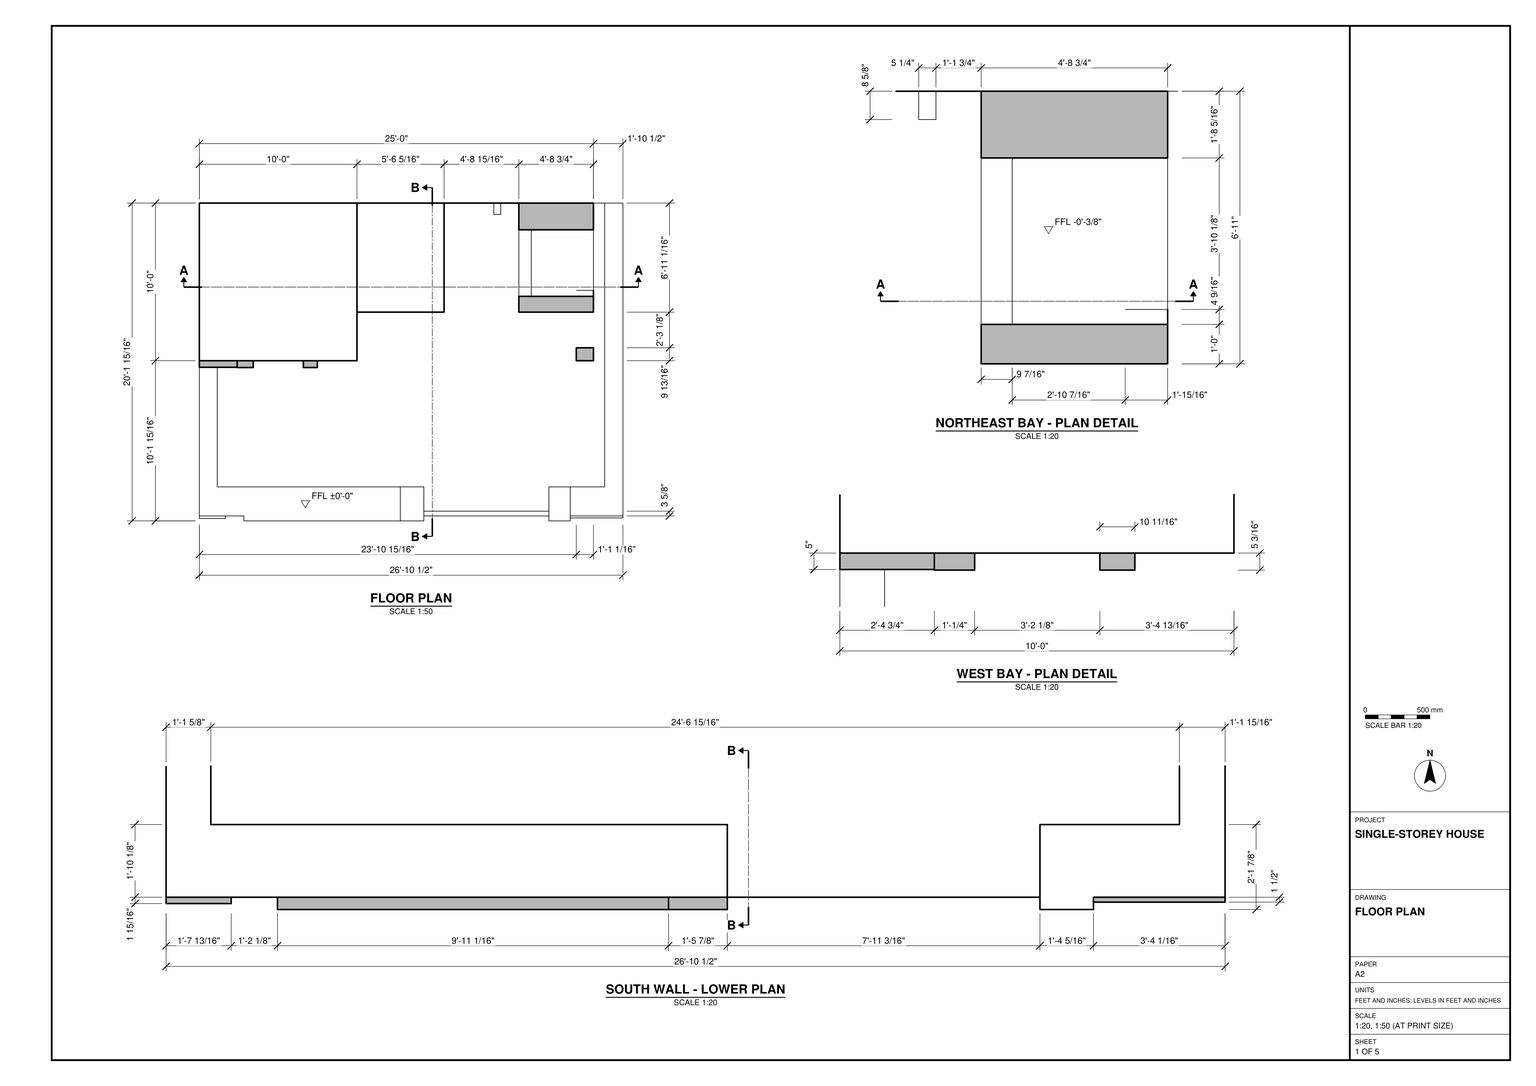
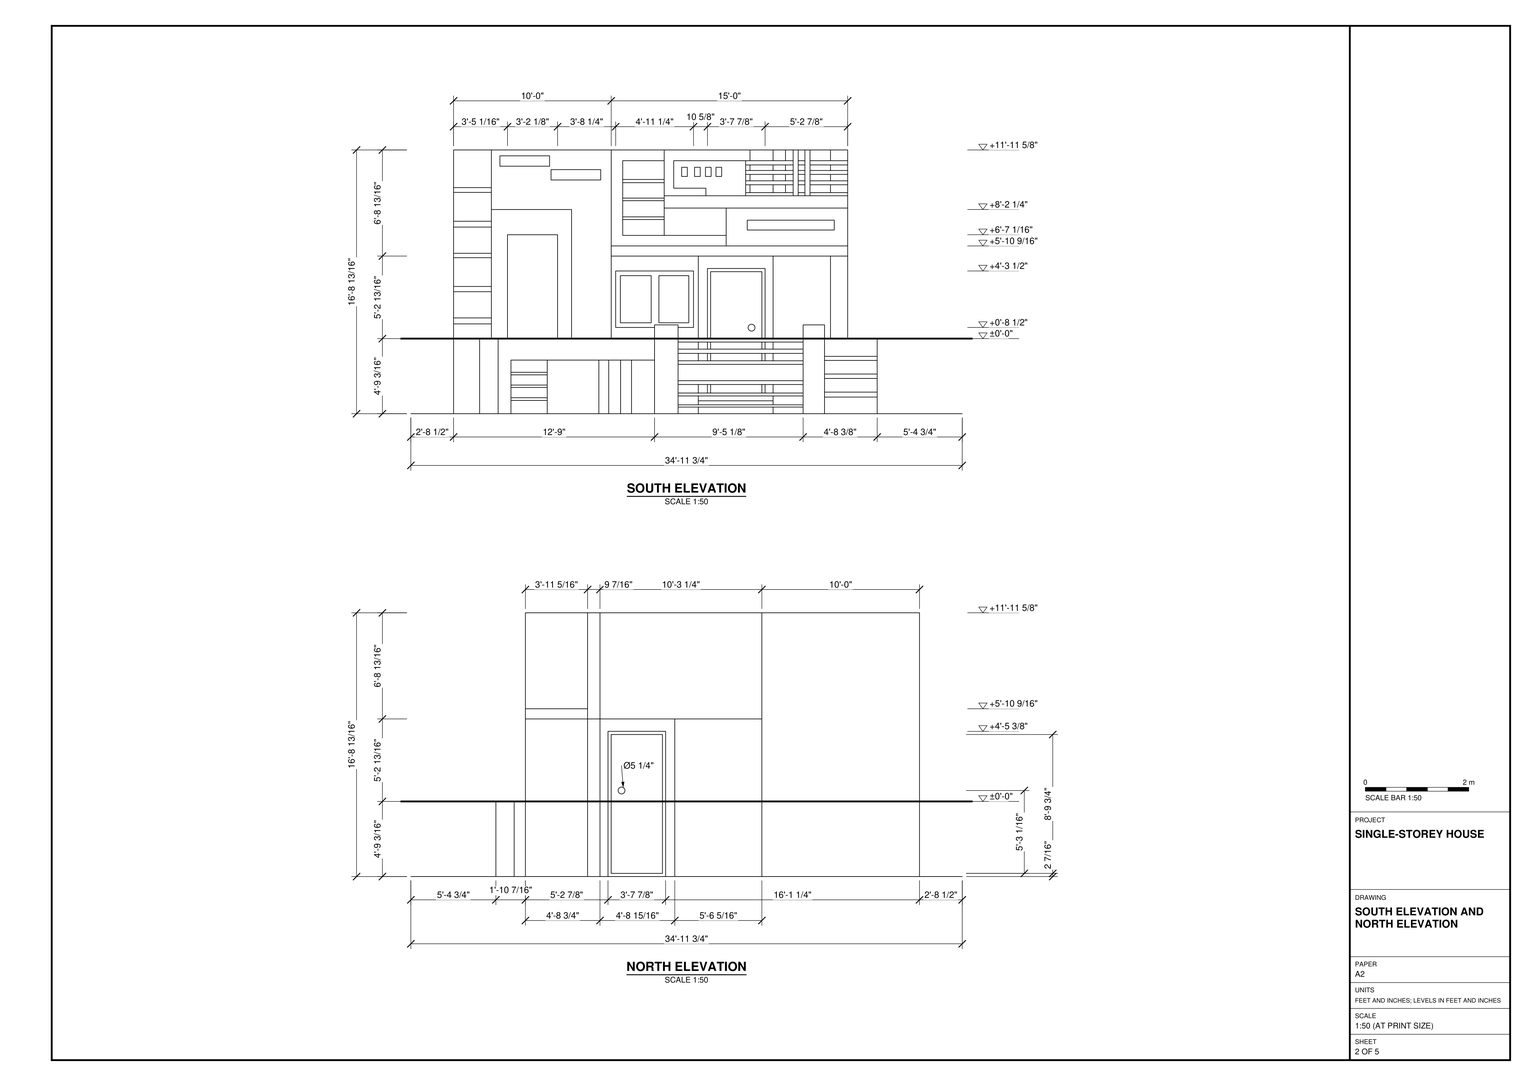
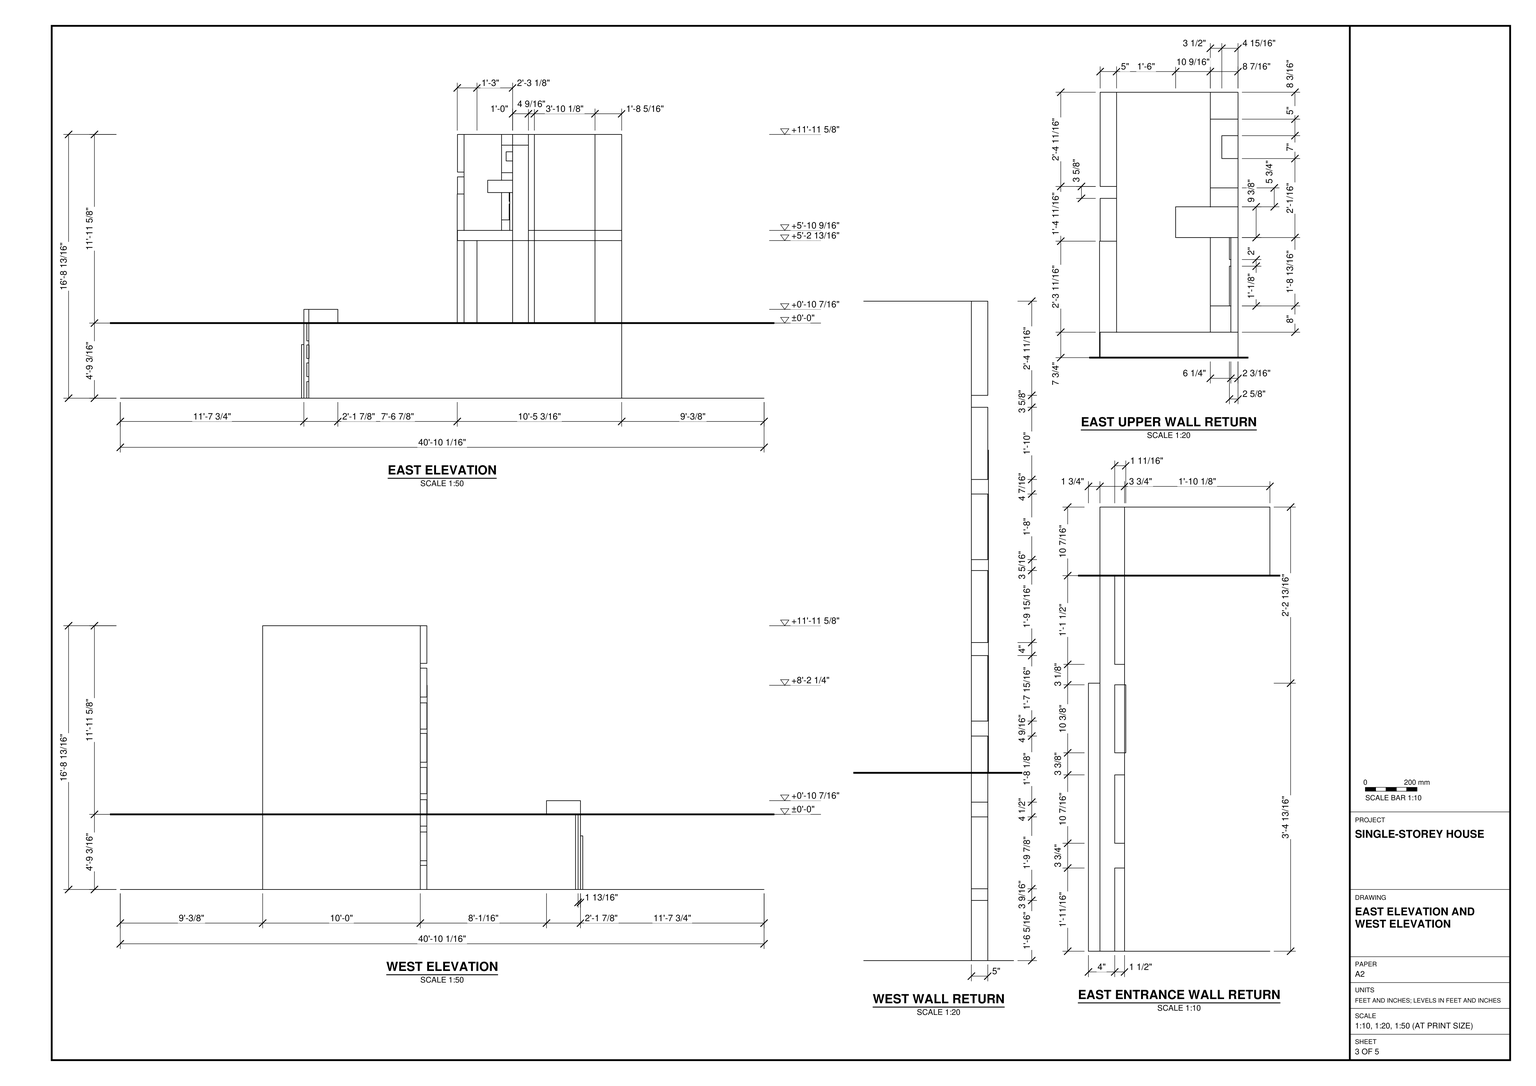
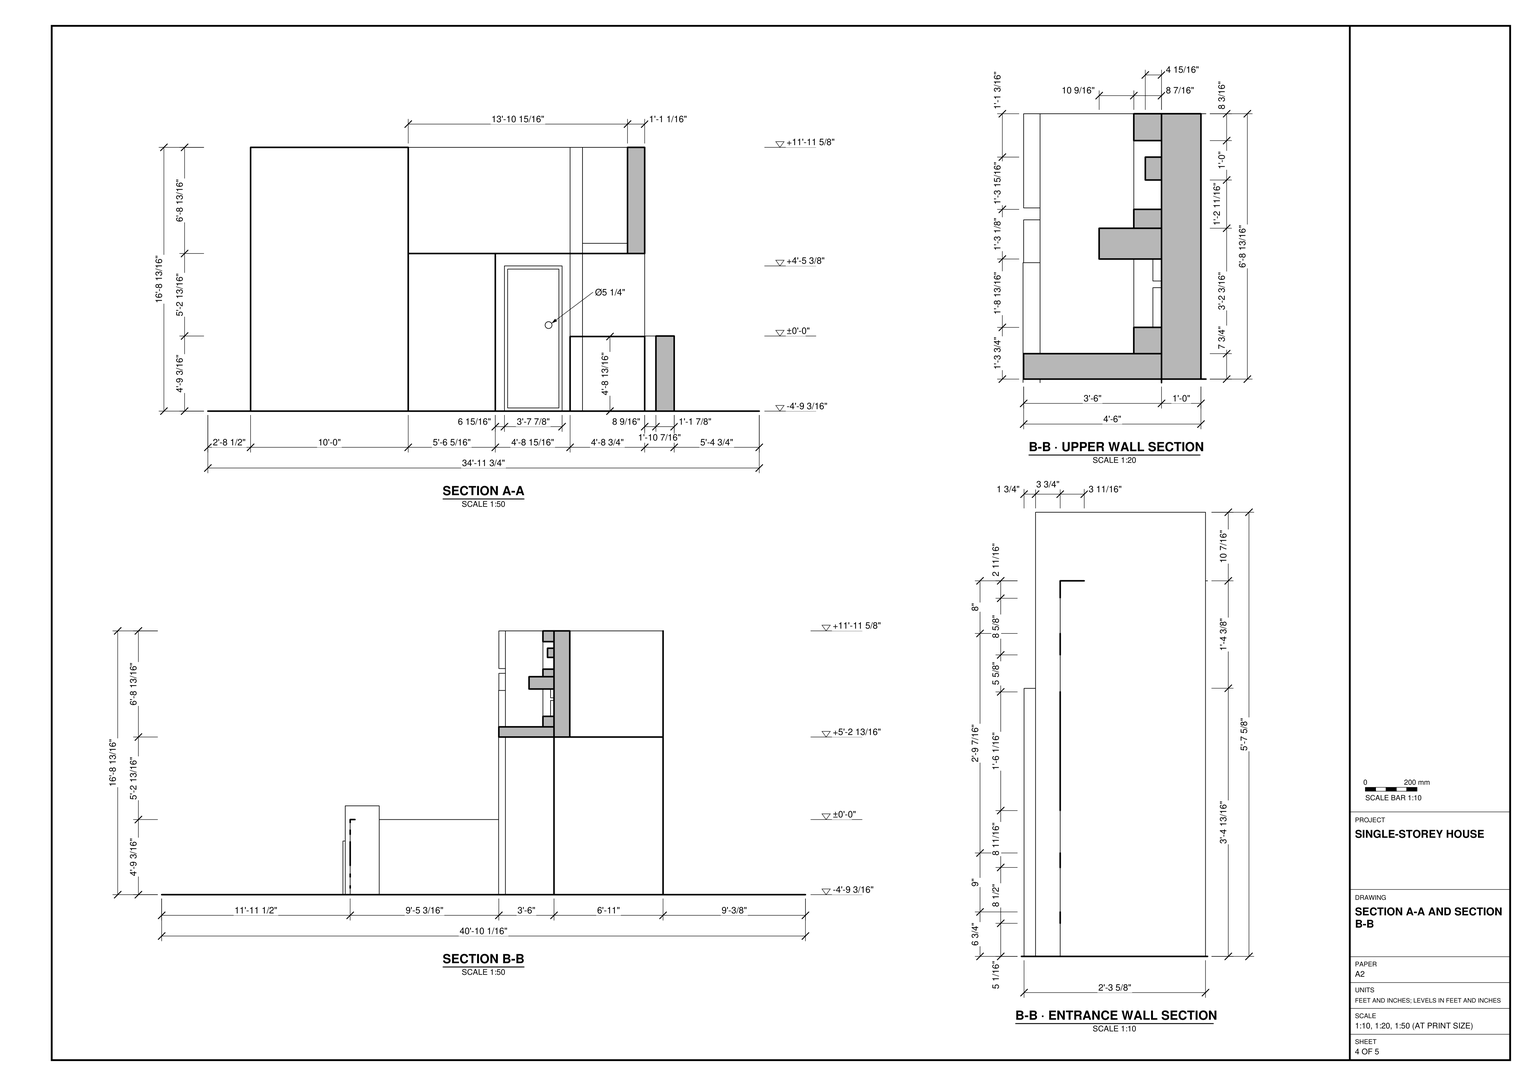
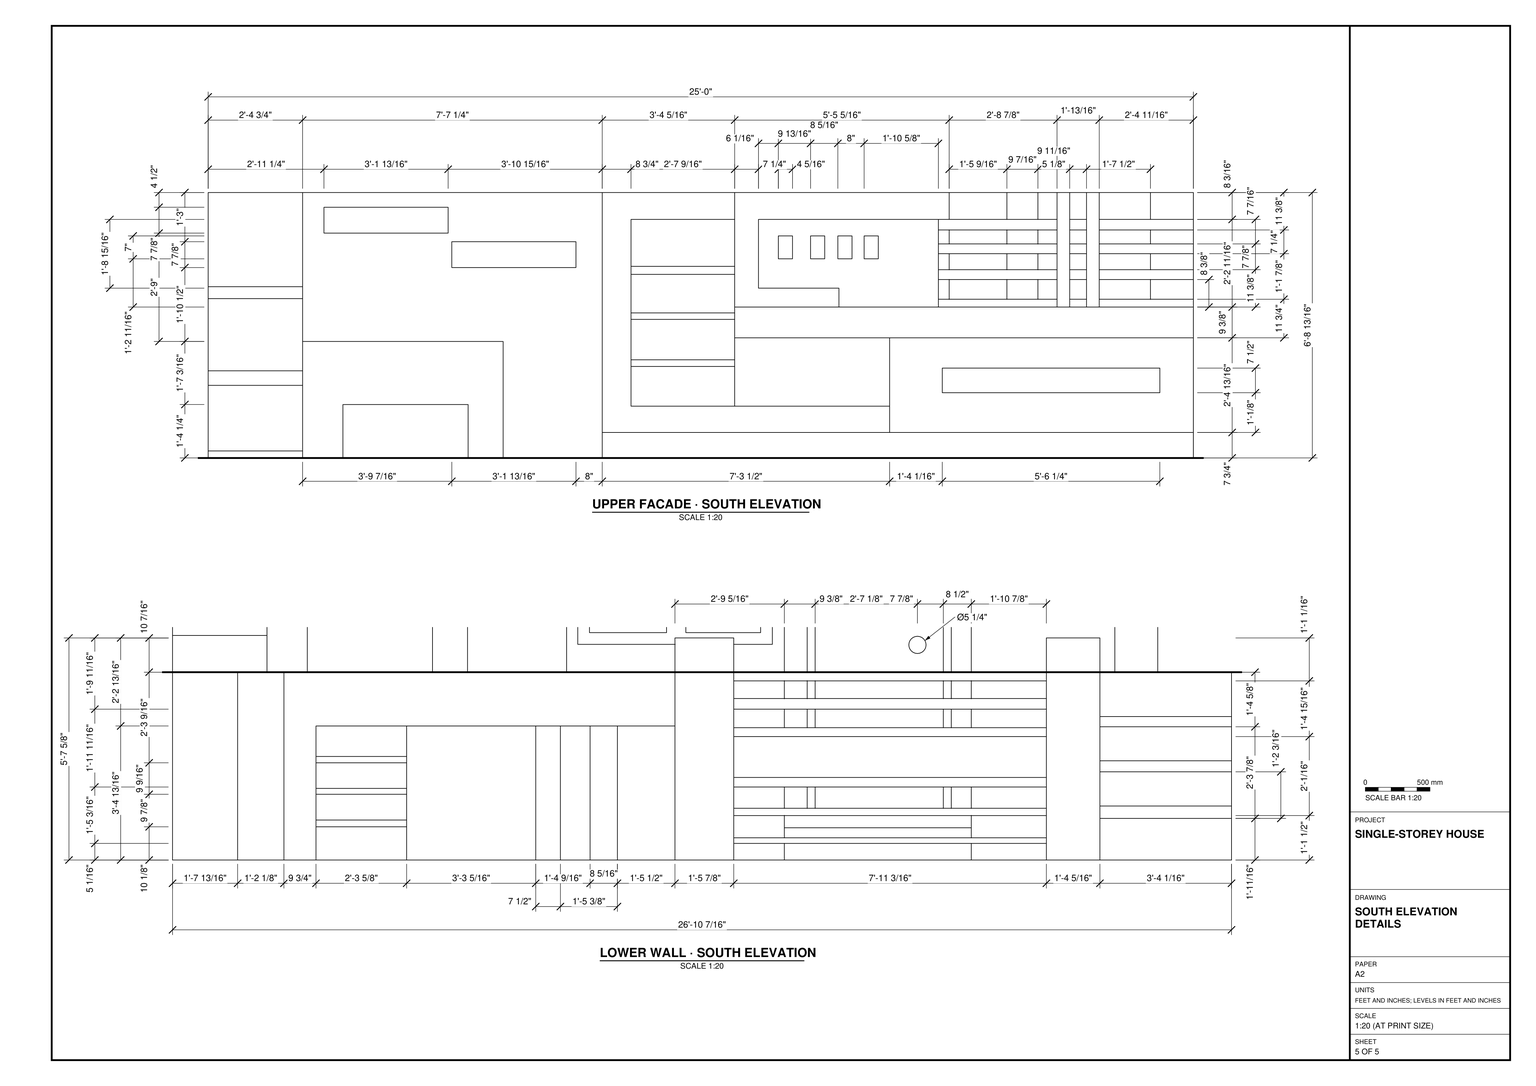
Build the single-storey house in SketchUp from task_files/diagram_01.pdf. Work in feet and inches. The complete model measures 34'-11 3/4" along X, 40'-10 1/16" along Y and 16'-8 13/16" along Z. Use ±0'-0" as the finished floor level. The overall height includes geometry below this datum; it is not the height of the wall above the floor.

Set out the square west bay, the shallower adjoining bay and the narrow northeast bay from the floor plan. Leave the forecourt between the house and the south entrance wall. Follow the plan details for wall thicknesses and returns, and match the slab and roof edges to the drawings. On the south facade, place the divided window beside the entrance door. Model the tall rectangular framing on the west side and the bands and panels above the openings on the east side. Use the side elevations to determine how far these details project. Build the lower entrance wall with its posts and horizontal slats.

Keep the walls, slabs and roof separate as groups or components. Keep each furniture or joinery piece shown separate and use components for repeated parts. Any decor or loose items shown may be represented by suitable library components. Save one SketchUp model as output_files/single_storey_house_and_its_south_entrance_wall.skp.

# SketchUp Ruby script. Lengths in inches.
U = 1.inch
M = Sketchup.active_model
def pt(a) = Geom::Point3d.new(a.map { |v| v * U })
def face(e, loops, mat)
  f = e.add_face(loops[0].map { |a| pt(a) })
  loops[1..].each { |l| e.add_face(l.map { |a| pt(a) }).erase! }
  f.material = f.back_material = mat if mat
  f
end
# faces: each face lists its corners as indices into pts; further lists are holes
def faces(e, pts, list, mat = nil) = list.each { |f| face(e, (f[0].is_a?(Array) ? f : [f]).map { |l| l.map { |i| pts[i] } }, mat) }
# xy, xz, yz: faces in a plane at the given z, y or x. An outline is a flat list of corners, or four numbers for a rectangle; further outlines are holes
def ring(l) = l.size == 4 ? [[l[0], l[1]], [l[2], l[1]], [l[2], l[3]], [l[0], l[3]]] : l.each_slice(2).to_a
def flat(e, list, mat, &to3) = list.each { |f| face(e, (f[0].is_a?(Array) ? f : [f]).map { |l| ring(l).map { |u, v| to3.(u, v) } }, mat) }
def xy(e, z, list, mat = nil) = flat(e, list, mat) { |x, y| [x, y, z] }
def xz(e, y, list, mat = nil) = flat(e, list, mat) { |x, z| [x, y, z] }
def yz(e, x, list, mat = nil) = flat(e, list, mat) { |y, z| [x, y, z] }
def lines(e, pts, list) = list.each { |a, b| e.add_line(pt(pts[a]), pt(pts[b])) }
# prism: a flat outline (further loops are holes) pulled along v
def prism(e, loops, v, mat = nil)
  f = face(e, loops, mat); d = Geom::Vector3d.new(v.map { |x| x * U })
  f.pushpull(f.normal.samedirection?(d) ? d.length : -d.length)
end
def box(e, o, s, mat = nil) = prism(e, [[o, [o[0] + s[0], o[1], o[2]], [o[0] + s[0], o[1] + s[1], o[2]], [o[0], o[1] + s[1], o[2]]]], [0, 0, s[2]], mat)
def at(x, y, z, deg = 0) = Geom::Transformation.translation(pt([x, y, z])) * Geom::Transformation.rotation(ORIGIN, Z_AXIS, deg.degrees)
def axes(o, x, y, z) = Geom::Transformation.new([*x, 0, *y, 0, *z, 0, *pt(o).to_a, 1])
def part(name) = M.definitions.add(name)
# library, detail: a bought-in or finely detailed component or shape, given as its bounding box
def library(name, o, s) = part(name).tap { |d| box(d.entities, o, s) }
def detail(e, o, s) = box(e.add_group.entities, o, s)
def put(e, d, t, mat = nil) = e.add_instance(d, t).tap { |i| i.material = mat if mat }
def group(e, t, mat = nil) = e.add_group.tap { |g| g.transformation = t; g.material = mat if mat }.entities
root = M.entities
M.materials.add("[0006_Pink]").color = [255, 192, 203]
M.materials.add("[0017_IndianRed]").color = [205, 92, 92]
M.materials.add("[0063_GreenYellow]").color = [173, 255, 47]
M.materials.add("[0087_Cyan]").color = [0, 255, 255]
M.materials.add("[0108_Indigo]").color = [75, 0, 130]
M.materials.add("[0110_LightSlateGray]").color = [119, 136, 153]
M.materials.add("[0119_RosyBrown]").color = [188, 143, 143]
M.materials.add("[Brick Colored Blue]1").color = [144, 143, 146]
M.materials.add("[Metal Seamed]").color = [118, 119, 115]
M.materials.add("[Translucent Glass Gray]").color = [128, 128, 128]
M.materials["[Translucent Glass Gray]"].alpha = 0.5
M.materials.add("[Wood Lumber ButtJoined]").color = [164, 152, 112]
M.materials.add("[Wood Veneer 01]").color = [120, 70, 37]
xy(root,0,[[203.42,123.43,298.62,143.5],[143.13,138,150.63,143.5],[159.68,138,167.99,143.5],[66.45,139.75,76.21,143.5],[185.52,139.75,203.42,143.5],
  [298.62,139.75,314.92,143.5],[76.21,141.125,103.82,143.5],[32.53,141.5625,52.35,143.5],[314.92,142,354.99,143.5],[32.53,143.5,32.53,256.6875,46.15,256.6875,46.15,165.625,203.42,165.625,203.42,143.5],
  [203.42,143.5,203.42,165.625,46.15,165.625,46.15,256.6875,61.29,256.6875,61.29,256.5,73.57,256.5,73.57,261.6875,111.69,261.6875,111.69,256.5,122.36,256.5,122.36,261.6875,152.53,261.6875,152.53,298.67,218.83,298.67,218.83,244.42,275.75,244.42,275.75,298.67,332.53,298.67,332.53,271.53,319.47,271.53,319.47,261.6875,332.53,261.6875,332.53,381.6875,341.09,381.6875,341.09,165.625,298.62,165.625,298.62,143.5],[298.62,143.5,298.62,165.625,341.09,165.625,341.09,381.6875,354.99,381.6875,354.99,143.5],[218.83,244.42,275.75,261.61],[61.29,256.5,73.57,261.6875],[111.69,256.5,122.36,261.6875],
  [32.53,256.6875,46.15,261.6875],[46.15,256.6875,61.29,261.6875],[218.83,261.61,275.75,278.81],[32.53,261.6875,152.53,381.6875],[319.47,261.6875,332.53,271.53],
  [218.83,278.81,275.75,298.67],[152.53,298.67,218.83,381.6875],[218.83,298.67,275.75,381.6875],[275.75,298.67,285.2,381.6875],[285.2,298.67,285.2,381.6875,332.53,381.6875,332.53,315.23,319.47,315.23,319.47,298.67],
  [319.47,298.67,332.53,315.23]])
xy(root,0,[[[0,0,419.74,490.0625],[218.83,244.42,275.75,244.42,275.75,298.67,332.53,298.67,332.53,381.6875,32.53,381.6875,32.53,256.6875,61.29,256.6875,61.29,256.5,73.57,256.5,73.57,261.6875,111.69,261.6875,111.69,256.5,122.36,256.5,122.36,261.6875,152.53,261.6875,152.53,298.67,218.83,298.67],[203.42,123.43,298.62,123.43,298.62,139.75,314.92,139.75,314.92,142,354.99,142,354.99,381.6875,341.09,381.6875,341.09,165.625,298.62,165.625,298.62,143.5,185.52,143.5,185.52,139.75,203.42,139.75],[319.47,261.6875,332.53,271.53],[66.45,139.75,76.21,139.75,76.21,141.125,103.82,141.125,103.82,143.5,66.45,143.5],[159.68,138,167.99,143.5],[143.13,138,150.63,143.5],[32.53,141.5625,52.35,143.5]]],"[Brick Colored Blue]1")
xy(root,5.5,[[218.83,244.42,275.75,261.61]])
xy(root,9.8125,[[218.83,261.61,275.75,278.81]])
xy(root,10.11,[[76.21,141.125,103.82,143.5]])
xy(root,12.17,[[76.21,141.125,103.82,143.5]])
xy(root,12.67,[[314.92,142,354.99,143.5]])
xy(root,14.375,[[218.83,278.81,275.75,298.67]])
xy(root,16.4375,[[314.92,142,354.99,143.5]])
xy(root,18.33,[[32.53,256.6875,61.29,261.6875]])
xy(root,20.01,[[76.21,141.125,103.82,143.5]])
xy(root,21.8,[[76.21,141.125,103.82,143.5]])
xy(root,21.88,[[32.53,256.6875,61.29,261.6875]])
xy(root,26.85,[[314.92,142,354.99,143.5]])
xy(root,29.6,[[76.21,141.125,103.82,143.5]])
xy(root,30.21,[[314.92,142,354.99,143.5],[314.92,143.5,354.99,143.6875]])
xy(root,31.53,[[76.21,141.125,103.82,143.5]])
xy(root,40.57,[[314.92,142,354.99,143.5],[314.92,143.5,354.99,143.6875]])
xy(root,40.8125,[[143.13,138,150.63,139.75],[159.68,138,167.99,139.75],[143.13,139.75,150.63,143.5],[159.68,139.75,167.99,143.5],[76.21,141.125,103.82,143.5]])
xy(root,40.8125,[[76.21,139.75,103.82,141.125],[103.82,139.75,143.13,143.5],[150.63,139.75,159.68,143.5],[167.99,139.75,185.52,143.5]],"[0087_Cyan]")
xy(root,43.68,[[314.92,142,354.99,143.5]])
xy(root,43.77,[[32.53,256.6875,61.29,261.6875]])
xy(root,48.26,[[32.53,256.6875,61.29,261.6875]])
xy(root,56.8125,[[275.75,310.68,285.2,361.37],[285.2,310.68,332.53,361.37]],"[0006_Pink]")
xy(root,57.1875,[[66.45,139.75,185.52,143.5],[314.92,142,354.99,143.5],[32.53,143.5,185.52,143.5,185.52,165.625,46.15,165.625,46.15,256.6875,32.53,256.6875],[314.92,143.5,354.99,143.5,354.99,381.6875,341.09,381.6875,341.09,165.625,314.92,165.625]])
xy(root,57.1875,[[32.53,141.5625,52.35,143.5]],"[0108_Indigo]")
xy(root,57.1875,[[203.42,143.5,298.62,147.15]],"[Metal Seamed]")
xy(root,67.625,[[185.52,139.75,203.42,143.5],[298.62,139.75,314.92,165.625],[185.52,143.5,203.42,165.625]],"[0108_Indigo]")
xy(root,68.38,[[32.53,256.6875,61.29,261.6875]])
xy(root,72.95,[[32.53,256.6875,61.29,261.6875]])
xy(root,92.9,[[32.53,256.6875,61.29,261.6875]])
xy(root,96.87,[[32.53,256.6875,61.29,261.6875]])
xy(root,118.79,[[32.53,256.6875,61.29,261.6875]])
xy(root,120,[[319.47,261.6875,332.53,271.53],[152.53,298.67,218.83,310.68],[275.75,298.67,285.2,310.68],[285.2,298.67,319.47,310.68],[319.47,298.67,332.53,310.68],
  [152.53,310.68,218.83,381.6875],[319.47,310.68,332.53,361.37],[275.75,361.37,285.2,381.6875],[285.2,361.37,332.53,381.6875]])
xy(root,120,[[152.53,256.67,152.53,298.67,332.53,298.67,332.53,271.53,319.47,271.53,319.47,261.6875,332.53,261.6875,332.53,256.67],[218.83,298.67,275.75,310.68],[218.83,310.68,218.83,381.6875,275.75,381.6875,275.75,361.37,319.47,361.37,319.47,310.68]],"[0006_Pink]")
xy(root,122.12,[[32.53,256.6875,61.29,261.6875]])
xy(root,127.74,[[152.53,256.67,332.53,256.67,332.53,296.48,240.04,296.48,240.04,290.23,152.53,290.23],[152.53,290.23,218.83,298.67],[218.83,290.23,240.04,298.67],[240.04,296.48,275.75,298.67],[275.75,296.48,285.2,298.67],
  [285.2,296.48,332.53,298.67],[285.2,361.37,332.53,381.6875]])
xy(root,135.75,[[161.29,296.04,192.86,298.67]])
xy(root,135.75,[[161.29,290.23,192.86,296.04],[192.86,290.23,240.04,298.67]],"[0108_Indigo]")
xy(root,136.25,[[73.57,256.5,111.69,261.6875]],"[0108_Indigo]")
xy(root,139.85,[[256.08,296.48,322.33,298.67]])
xy(root,142.09,[[32.53,256.6875,61.29,261.6875]])
xy(root,146.52,[[32.53,256.6875,61.29,261.6875]])
xy(root,147.35,[[256.08,296.48,322.33,298.67]])
xy(root,147.84,[[161.29,296.04,192.86,298.67]])
xy(root,149.875,[[161.29,296.04,192.86,298.67]])
xy(root,155.45,[[61.29,256.5,122.36,261.6875]],"[0108_Indigo]")
xy(root,156.5625,[[240.04,296.48,332.53,298.67]])
xy(root,156.5625,[[192.86,279.67,192.86,298.67,240.04,298.67,240.04,296.48,332.53,296.48,332.53,279.67]],"[0108_Indigo]")
xy(root,162.18,[[161.29,296.04,192.86,298.67]])
xy(root,164.15,[[161.29,296.04,192.86,298.67]])
xy(root,165.9375,[[192.86,290.23,224.61,298.67]])
xy(root,165.9375,[[192.86,279.67,332.53,279.67,332.53,298.67,224.61,298.67,224.61,290.23,192.86,290.23]],"[0108_Indigo]")
xy(root,168.5,[[32.53,256.6875,61.29,261.6875]])
xy(root,171.6875,[[200.11,290.23,224.61,298.67]],"[0087_Cyan]")
xy(root,172.13,[[32.53,256.6875,61.29,261.6875]])
xy(root,175.89,[[161.29,296.04,192.86,298.67]])
xy(root,177.96,[[106.72,261.6875,144.53,267.0625]],"[0087_Cyan]")
xy(root,178.33,[[161.29,296.04,192.86,298.67]])
xy(root,180.62,[[206.15,293.73,210.46,298.67],[215.96,293.73,220.28,298.67],[224.28,293.73,228.59,298.67],[232.28,293.73,236.59,298.67]],"[0108_Indigo]")
xy(root,185.83,[[106.72,261.6875,144.53,267.0625]],"[0087_Cyan]")
xy(root,187.6,[[206.15,293.73,210.46,298.67],[215.96,293.73,220.28,298.67],[224.28,293.73,228.59,298.67],[232.28,293.73,236.59,298.67]],"[0108_Indigo]")
xy(root,188.45,[[67.79,261.6875,105.61,268.1875]],"[0087_Cyan]")
xy(root,192.625,[[161.29,296.04,192.86,298.67],[258.17,298.67,291.02,310.68],[294.875,298.67,299.99,310.68],[303.86,298.67,332.53,310.68]])
xy(root,192.625,[[200.11,290.23,254.89,298.67],[254.89,290.23,258.17,298.67]],"[0087_Cyan]")
xy(root,192.625,[[161.29,290.23,192.86,296.04]],"[0108_Indigo]")
xy(root,196.32,[[67.79,261.6875,105.61,268.1875]],"[0087_Cyan]")
xy(root,200.8125,[[32.53,256.6875,61.29,261.6875],[32.53,261.6875,152.53,381.6875],[152.53,290.23,192.86,298.67],[152.53,298.67,258.17,310.68]])
xy(root,200.8125,[[291.02,298.67,294.875,310.68],[299.99,298.67,303.86,310.68],[319.47,310.68,332.53,361.37]],"[0063_GreenYellow]")
xy(root,200.8125,[[192.86,290.23,258.17,298.67]],"[0087_Cyan]")
xz(root,138,[[143.13,0,150.63,40.8125],[159.68,0,167.99,40.8125]],"[0108_Indigo]")
xz(root,139.75,[[66.45,0,76.21,0,76.21,40.8125,185.52,40.8125,185.52,57.1875,66.45,57.1875]],"[0087_Cyan]")
xz(root,139.75,[[185.52,0,203.42,67.625],[298.62,0,314.92,67.625]],"[0108_Indigo]")
xz(root,141.125,[[76.21,0,103.82,10.11],[76.21,12.17,103.82,20.01],[76.21,21.8,103.82,29.6],[76.21,31.53,103.82,40.8125]],"[0063_GreenYellow]")
xz(root,141.5625,[[32.53,0,52.35,57.1875]],"[0108_Indigo]")
xz(root,142,[[314.92,0,354.99,12.67],[314.92,16.4375,354.99,26.85],[314.92,30.21,354.99,40.57],[314.92,43.68,354.99,57.1875]],"[0063_GreenYellow]")
xz(root,143.5,[[32.53,0,52.35,57.1875],[52.35,0,66.45,57.1875],[66.45,0,66.45,57.1875,185.52,57.1875,185.52,40.8125,76.21,40.8125,76.21,0],[76.21,0,103.82,10.11],[103.82,0,143.13,40.8125],
  [143.13,0,150.63,40.8125],[150.63,0,159.68,40.8125],[159.68,0,167.99,40.8125],[167.99,0,185.52,40.8125],[185.52,0,203.42,67.625],
  [314.92,0,354.99,12.67],[76.21,10.11,103.82,12.17],[76.21,12.17,103.82,20.01],[314.92,12.67,354.99,16.4375],[314.92,16.4375,354.99,26.85],
  [76.21,20.01,103.82,21.8],[76.21,21.8,103.82,29.6],[314.92,26.85,354.99,30.21],[76.21,29.6,103.82,31.53],[314.92,30.21,354.99,40.57],
  [76.21,31.53,103.82,40.8125],[314.92,40.57,354.99,43.68],[314.92,43.68,354.99,57.1875]])
xz(root,143.5,[[203.42,5.05,298.62,6.76],[203.42,13.53,298.62,15.75],[203.42,22.22,298.62,25.13],[203.42,25.13,298.62,37.58],[203.42,37.58,298.62,40.29],
  [203.42,45.93,298.62,49.17],[203.42,54.54,298.62,57.1875]],"[Metal Seamed]")
xz(root,143.6875,[[314.92,30.21,354.99,40.57]])
xz(root,165.625,[[46.15,0,185.52,57.1875],[314.92,0,341.09,57.1875]])
xz(root,165.625,[[185.52,0,203.42,57.1875],[298.62,0,314.92,57.1875],[185.52,57.1875,203.42,67.625],[298.62,57.1875,314.92,67.625]],"[0108_Indigo]")
xz(root,244.42,[[218.83,0,275.75,5.5]])
xz(root,256.5,[[61.29,0,73.57,0,73.57,136.25,111.69,136.25,111.69,0,122.36,0,122.36,155.45,61.29,155.45]],"[0108_Indigo]")
xz(root,256.67,[[152.53,120,332.53,127.74]])
xz(root,256.6875,[[32.53,0,46.15,18.33],[32.53,18.33,46.15,21.88],[32.53,21.88,46.15,43.77],[32.53,43.77,46.15,48.26],[32.53,48.26,46.15,57.1875]])
xz(root,256.6875,[[46.15,0,61.29,18.33],[46.15,21.88,61.29,43.77],[46.15,48.26,61.29,48.26,61.29,68.38,32.53,68.38,32.53,57.1875,46.15,57.1875],[32.53,72.95,61.29,92.9],[32.53,96.87,61.29,118.79],
  [32.53,122.12,61.29,142.09],[32.53,146.52,61.29,168.5],[32.53,172.13,61.29,200.8125]],"[0063_GreenYellow]")
xz(root,261.61,[[218.83,0,275.75,5.5],[218.83,5.5,275.75,9.8125]])
xz(root,261.6875,[[32.53,0,61.29,18.33],[61.29,0,61.29,155.45,122.36,155.45,122.36,0,111.69,0,111.69,136.25,73.57,136.25,73.57,0],[32.53,18.33,61.29,21.88],[32.53,21.88,61.29,43.77],[32.53,43.77,61.29,48.26],
  [32.53,48.26,61.29,68.38],[32.53,68.38,61.29,72.95],[32.53,72.95,61.29,92.9],[32.53,92.9,61.29,96.87],[32.53,96.87,61.29,118.79],
  [32.53,118.79,61.29,122.12],[32.53,122.12,61.29,142.09],[32.53,142.09,61.29,146.52],[32.53,146.52,61.29,168.5],[32.53,168.5,61.29,172.13],
  [32.53,172.13,61.29,200.8125]])
xz(root,261.6875,[[319.47,0,332.53,120]],"[0006_Pink]")
xz(root,261.6875,[[[122.36,0,152.53,0,152.53,200.8125,61.29,200.8125,61.29,155.45,122.36,155.45],[106.72,177.96,144.53,185.83],[67.79,188.45,105.61,196.32]]],"[0119_RosyBrown]")
xz(root,261.6875,[[73.57,0,111.69,136.25]],"[Translucent Glass Gray]")
xz(root,267.0625,[[106.72,177.96,144.53,185.83]],"[0087_Cyan]")
xz(root,268.1875,[[67.79,188.45,105.61,196.32]],"[0087_Cyan]")
xz(root,271.53,[[319.47,0,332.53,120]])
xz(root,278.81,[[218.83,0,275.75,9.8125],[218.83,9.8125,275.75,14.375]])
xz(root,279.67,[[192.86,156.5625,332.53,165.9375]],"[0108_Indigo]")
xz(root,290.23,[[192.86,165.9375,224.61,165.9375,224.61,171.6875,200.11,171.6875,200.11,192.625,258.17,192.625,258.17,200.8125,192.86,200.8125]],"[0087_Cyan]")
xz(root,290.23,[[152.53,127.74,240.04,127.74,240.04,135.75,161.29,135.75,161.29,192.625,192.86,192.625,192.86,200.8125,152.53,200.8125]],"[0108_Indigo]")
xz(root,293.73,[[206.15,180.62,210.46,187.6],[215.96,180.62,220.28,187.6],[224.28,180.62,228.59,187.6],[232.28,180.62,236.59,187.6]],"[0108_Indigo]")
xz(root,296.04,[[161.29,135.75,192.86,147.84],[161.29,149.875,192.86,162.18],[161.29,164.15,192.86,175.89],[161.29,178.33,192.86,192.625]],"[0063_GreenYellow]")
xz(root,296.48,[[[240.04,127.74,332.53,156.5625],[256.08,139.85,322.33,147.35]]],"[0119_RosyBrown]")
xz(root,298.67,[[218.83,0,275.75,14.375],[152.53,120,218.83,127.74],[218.83,120,275.75,127.74],[275.75,120,285.2,127.74],[285.2,120,332.53,127.74],
  [152.53,127.74,152.53,200.8125,192.86,200.8125,192.86,192.625,161.29,192.625,161.29,135.75,240.04,135.75,240.04,127.74],[[240.04,127.74,332.53,156.5625],[256.08,139.85,322.33,147.35]],[161.29,135.75,192.86,147.84],[256.08,139.85,322.33,147.35],[161.29,147.84,192.86,149.875],
  [161.29,149.875,192.86,162.18],[192.86,156.5625,332.53,165.9375],[161.29,162.18,192.86,164.15],[161.29,164.15,192.86,175.89],[192.86,165.9375,192.86,200.8125,258.17,200.8125,258.17,192.625,200.11,192.625,200.11,171.6875,224.61,171.6875,224.61,165.9375],
  [[224.61,165.9375,254.89,165.9375,254.89,192.625,200.11,192.625,200.11,171.6875,224.61,171.6875],[206.15,180.62,210.46,187.6],[215.96,180.62,220.28,187.6],[224.28,180.62,228.59,187.6],[232.28,180.62,236.59,187.6]],[161.29,175.89,192.86,178.33],[161.29,178.33,192.86,192.625],[206.15,180.62,210.46,187.6],[215.96,180.62,220.28,187.6],
  [224.28,180.62,228.59,187.6],[232.28,180.62,236.59,187.6]])
xz(root,298.67,[[[152.53,0,218.83,120],[155.92,65.67,215.17,108.67]],[275.75,0,332.53,120]],"[0006_Pink]")
xz(root,298.67,[[291.02,165.9375,294.875,200.8125],[299.99,165.9375,303.86,200.8125]],"[0063_GreenYellow]")
xz(root,298.67,[[192.86,135.75,240.04,156.5625]],"[0110_LightSlateGray]")
xz(root,298.67,[[254.89,165.9375,291.02,168.32],[294.875,165.9375,299.99,168.32],[303.86,165.9375,332.53,168.32],[254.89,174.3125,291.02,177.3125],[294.875,174.3125,299.99,177.3125],
  [303.86,174.3125,332.53,177.3125],[254.89,182.1875,291.02,185.17],[294.875,182.1875,299.99,185.17],[303.86,182.1875,332.53,185.17],[254.89,189.41,291.02,192.625],
  [294.875,189.41,299.99,192.625],[303.86,189.41,332.53,192.625]],"[Metal Seamed]")
xz(root,298.67,[[159.49,69.24,182.96,105.1],[188.83,69.24,211.61,105.1]],"[Translucent Glass Gray]")
xz(root,298.67,[[[155.92,65.67,215.17,108.67],[159.49,69.24,182.96,105.1],[188.83,69.24,211.61,105.1]]],"[Wood Veneer 01]")
xz(root,310.68,[[275.75,56.8125,285.2,120],[152.53,120,258.17,192.625],[258.17,120,319.47,161.72],[319.47,120,332.53,161.72],[152.53,192.625,258.17,200.8125]])
xz(root,310.68,[[285.2,56.8125,332.53,120]],"[0006_Pink]")
xz(root,310.68,[[319.47,161.72,332.53,192.625],[291.02,192.625,294.875,200.8125],[299.99,192.625,303.86,200.8125],[319.47,192.625,332.53,200.8125]],"[0063_GreenYellow]")
xz(root,361.37,[[285.2,120,319.47,127.74],[319.47,120,332.53,127.74],[319.47,127.74,332.53,200.8125]])
xz(root,361.37,[[275.75,56.8125,285.2,120],[285.2,56.8125,332.53,120]],"[0006_Pink]")
xz(root,373.0625,[[259.36,62.88,260.03,62.97,260.67,63.23,261.21,63.65,261.63,64.19,261.89,64.83,261.98,65.51,261.89,66.1875,261.63,66.82,261.21,67.36,260.67,67.78,260.03,68.04,259.36,68.13,258.68,68.04,258.04,67.78,257.5,67.36,257.08,66.82,256.82,66.1875,256.73,65.51,256.82,64.83,257.08,64.19,257.5,63.65,258.04,63.23,258.68,62.97]],"[Wood Lumber ButtJoined]")
xz(root,381.6875,[[32.53,0,152.53,200.8125],[152.53,0,218.83,120],[275.75,0,285.2,120],[285.2,0,332.53,120],[332.53,0,341.09,57.1875],
  [341.09,0,354.99,57.1875],[152.53,120,275.75,200.8125],[275.75,120,285.2,200.8125],[285.2,120,332.53,127.74],[285.2,127.74,332.53,200.8125]])
xz(root,381.6875,[[[225.78,0,269.66,110.5625],[228.2,2.42,267.24,108.14]]],"[0006_Pink]")
xz(root,381.6875,[[218.83,0,218.83,120,275.75,120,275.75,0,269.66,0,269.66,110.5625,225.78,110.5625,225.78,0]],"[Translucent Glass Gray]")
xz(root,381.6875,[[[228.2,2.42,267.24,108.14],[259.36,62.88,260.03,62.97,260.67,63.23,261.21,63.65,261.63,64.19,261.89,64.83,261.98,65.51,261.89,66.1875,261.63,66.82,261.21,67.36,260.67,67.78,260.03,68.04,259.36,68.13,258.68,68.04,258.04,67.78,257.5,67.36,257.08,66.82,256.82,66.1875,256.73,65.51,256.82,64.83,257.08,64.19,257.5,63.65,258.04,63.23,258.68,62.97]],[259.36,62.88,258.68,62.97,258.04,63.23,257.5,63.65,257.08,64.19,256.82,64.83,256.73,65.51,256.82,66.1875,257.08,66.82,257.5,67.36,258.04,67.78,258.68,68.04,259.36,68.13,260.03,68.04,260.67,67.78,261.21,67.36,261.63,66.82,261.89,66.1875,261.98,65.51,261.89,64.83,261.63,64.19,261.21,63.65,260.67,63.23,260.03,62.97]],"[Wood Veneer 01]")
yz(root,32.53,[[141.5625,0,143.5,57.1875],[143.5,0,256.6875,57.1875],[256.6875,0,261.6875,18.33],[261.6875,0,381.6875,200.8125],[256.6875,21.88,261.6875,43.77],
  [256.6875,48.26,261.6875,68.38],[256.6875,72.95,261.6875,92.9],[256.6875,96.87,261.6875,118.79],[256.6875,122.12,261.6875,142.09],[256.6875,146.52,261.6875,168.5],
  [256.6875,172.13,261.6875,200.8125]])
yz(root,46.15,[[165.625,0,256.6875,57.1875]])
yz(root,52.35,[[141.5625,0,143.5,57.1875]],"[0108_Indigo]")
yz(root,61.29,[[256.5,0,256.6875,18.33],[256.6875,0,261.6875,18.33],[256.5,18.33,261.6875,21.88],[256.5,21.88,256.6875,43.77],[256.6875,21.88,261.6875,43.77],
  [256.5,43.77,261.6875,48.26],[256.5,48.26,256.6875,68.38],[256.6875,48.26,261.6875,68.38],[256.5,68.38,261.6875,72.95],[256.5,72.95,256.6875,92.9],
  [256.6875,72.95,261.6875,92.9],[256.5,92.9,261.6875,96.87],[256.5,96.87,256.6875,118.79],[256.6875,96.87,261.6875,118.79],[256.5,118.79,261.6875,122.12],
  [256.5,122.12,256.6875,142.09],[256.6875,122.12,261.6875,142.09],[256.5,142.09,261.6875,146.52],[256.5,146.52,256.6875,155.45],[256.6875,146.52,261.6875,155.45],
  [256.6875,155.45,261.6875,168.5],[256.6875,172.13,261.6875,200.8125]])
yz(root,66.45,[[139.75,0,143.5,57.1875]],"[0087_Cyan]")
yz(root,67.79,[[261.6875,188.45,268.1875,196.32]],"[0087_Cyan]")
yz(root,73.57,[[256.5,0,261.6875,136.25]],"[0108_Indigo]")
yz(root,76.21,[[141.125,0,143.5,10.11],[141.125,12.17,143.5,20.01],[141.125,21.8,143.5,29.6],[141.125,31.53,143.5,40.8125]])
yz(root,76.21,[[139.75,0,141.125,10.11],[139.75,10.11,143.5,12.17],[139.75,12.17,141.125,20.01],[139.75,20.01,143.5,21.8],[139.75,21.8,141.125,29.6],
  [139.75,29.6,143.5,31.53],[139.75,31.53,141.125,40.8125]],"[0087_Cyan]")
yz(root,103.82,[[141.125,0,143.5,10.11],[141.125,12.17,143.5,20.01],[141.125,21.8,143.5,29.6],[141.125,31.53,143.5,40.8125]])
yz(root,105.61,[[261.6875,188.45,268.1875,196.32]],"[0087_Cyan]")
yz(root,106.72,[[261.6875,177.96,267.0625,185.83]],"[0087_Cyan]")
yz(root,111.69,[[256.5,0,261.6875,136.25]],"[0108_Indigo]")
yz(root,122.36,[[256.5,0,261.6875,155.45]],"[0108_Indigo]")
yz(root,143.13,[[138,0,143.5,40.8125]],"[0108_Indigo]")
yz(root,144.53,[[261.6875,177.96,267.0625,185.83]],"[0087_Cyan]")
yz(root,150.63,[[138,0,143.5,40.8125]],"[0108_Indigo]")
yz(root,152.53,[[298.67,0,381.6875,120],[256.67,120,261.6875,127.74],[261.6875,120,298.67,127.74],[298.67,120,310.68,192.625],[310.68,120,381.6875,200.8125],
  [290.23,127.74,298.67,192.625],[290.23,192.625,298.67,200.8125],[298.67,192.625,310.68,200.8125]])
yz(root,152.53,[[261.6875,0,298.67,120],[261.6875,127.74,290.23,200.8125]],"[0119_RosyBrown]")
yz(root,159.68,[[138,0,143.5,40.8125]],"[0108_Indigo]")
yz(root,161.29,[[296.04,135.75,298.67,147.84],[296.04,149.875,298.67,162.18],[296.04,164.15,298.67,175.89],[296.04,178.33,298.67,192.625]])
yz(root,161.29,[[290.23,135.75,296.04,135.75,296.04,147.84,298.67,147.84,298.67,149.875,296.04,149.875,296.04,162.18,298.67,162.18,298.67,164.15,296.04,164.15,296.04,175.89,298.67,175.89,298.67,178.33,296.04,178.33,296.04,192.625,290.23,192.625]],"[0108_Indigo]")
yz(root,167.99,[[138,0,143.5,40.8125]],"[0108_Indigo]")
yz(root,185.52,[[139.75,40.8125,143.5,57.1875]])
yz(root,185.52,[[139.75,0,143.5,40.8125],[139.75,57.1875,143.5,67.625],[143.5,57.1875,165.625,67.625]],"[0108_Indigo]")
yz(root,192.86,[[296.04,135.75,298.67,147.84],[296.04,149.875,298.67,156.5625],[296.04,156.5625,298.67,162.18],[296.04,164.15,298.67,165.9375],[290.23,165.9375,296.04,175.89],
  [296.04,165.9375,298.67,175.89],[290.23,175.89,298.67,178.33],[290.23,178.33,296.04,192.625],[296.04,178.33,298.67,192.625],[290.23,192.625,298.67,200.8125]])
yz(root,192.86,[[279.67,156.5625,296.04,162.18],[279.67,162.18,298.67,164.15],[279.67,164.15,296.04,165.9375]],"[0108_Indigo]")
yz(root,200.11,[[290.23,171.6875,298.67,192.625]],"[0087_Cyan]")
yz(root,203.42,[[139.75,0,143.5,5.05],[143.5,0,165.625,57.1875],[139.75,5.05,143.5,6.76],[139.75,6.76,143.5,13.53],[139.75,13.53,143.5,15.75],
  [139.75,15.75,143.5,22.22],[139.75,22.22,143.5,25.13],[139.75,25.13,143.5,37.58],[139.75,37.58,143.5,40.29],[139.75,40.29,143.5,45.93],
  [139.75,45.93,143.5,49.17],[139.75,49.17,143.5,54.54],[139.75,54.54,143.5,57.1875],[139.75,57.1875,143.5,67.625],[143.5,57.1875,147.15,67.625],
  [147.15,57.1875,165.625,67.625]],"[0108_Indigo]")
yz(root,206.15,[[293.73,180.62,298.67,187.6]],"[0108_Indigo]")
yz(root,210.46,[[293.73,180.62,298.67,187.6]],"[0108_Indigo]")
yz(root,215.96,[[293.73,180.62,298.67,187.6]],"[0108_Indigo]")
yz(root,218.83,[[244.42,0,261.61,5.5],[261.61,0,278.81,9.8125],[278.81,0,298.67,14.375]])
yz(root,218.83,[[298.67,0,381.6875,120]],"[0006_Pink]")
yz(root,220.28,[[293.73,180.62,298.67,187.6]],"[0108_Indigo]")
yz(root,224.28,[[293.73,180.62,298.67,187.6]],"[0108_Indigo]")
yz(root,224.61,[[290.23,165.9375,298.67,171.6875]],"[0087_Cyan]")
yz(root,228.59,[[293.73,180.62,298.67,187.6]],"[0108_Indigo]")
yz(root,232.28,[[293.73,180.62,298.67,187.6]],"[0108_Indigo]")
yz(root,236.59,[[293.73,180.62,298.67,187.6]],"[0108_Indigo]")
yz(root,240.04,[[296.48,127.74,298.67,135.75],[296.48,135.75,298.67,153.61],[296.48,153.61,298.67,156.5625]])
yz(root,240.04,[[290.23,127.74,296.48,135.75]],"[0108_Indigo]")
yz(root,256.08,[[296.48,139.85,298.67,147.35]])
yz(root,258.17,[[298.67,192.625,310.68,200.8125]])
yz(root,258.17,[[290.23,192.625,298.67,200.8125]],"[0087_Cyan]")
yz(root,275.75,[[244.42,0,261.61,5.5],[261.61,0,278.81,9.8125],[278.81,0,298.67,14.375]])
yz(root,275.75,[[298.67,0,298.67,120,310.68,120,310.68,56.8125,361.37,56.8125,361.37,120,381.6875,120,381.6875,0]],"[0006_Pink]")
yz(root,285.2,[[361.37,120,381.6875,127.74]])
yz(root,291.02,[[298.67,192.625,310.68,200.8125]],"[0063_GreenYellow]")
yz(root,294.875,[[298.67,192.625,310.68,200.8125]],"[0063_GreenYellow]")
yz(root,298.62,[[139.75,0,143.5,5.05],[143.5,0,143.5,40.29,139.75,40.29,139.75,67.625,165.625,67.625,165.625,0],[139.75,5.05,143.5,6.76],[139.75,6.76,143.5,13.53],[139.75,13.53,143.5,15.75],
  [139.75,15.75,143.5,22.22],[139.75,22.22,143.5,25.13],[139.75,25.13,143.5,37.58],[139.75,37.58,143.5,40.29]],"[0108_Indigo]")
yz(root,299.99,[[298.67,192.625,310.68,200.8125]],"[0063_GreenYellow]")
yz(root,303.86,[[298.67,192.625,310.68,200.8125]],"[0063_GreenYellow]")
yz(root,314.92,[[142,0,143.5,12.67],[142,16.4375,143.5,26.85],[142,30.21,143.5,40.57],[143.5,30.21,143.6875,40.57],[142,43.68,143.5,57.1875]])
yz(root,314.92,[[139.75,0,142,0,142,12.67,143.5,12.67,143.5,16.4375,142,16.4375,142,26.85,143.5,26.85,143.5,30.21,142,30.21,142,40.57,143.5,40.57,143.5,43.68,142,43.68,142,57.1875,143.5,57.1875,143.5,67.625,139.75,67.625],[143.5,57.1875,165.625,67.625]],"[0108_Indigo]")
yz(root,319.47,[[261.6875,0,271.53,120]])
yz(root,319.47,[[310.68,120,315.23,200.8125],[315.23,120,361.37,200.8125]],"[0063_GreenYellow]")
yz(root,322.33,[[296.48,139.85,298.67,147.35]])
yz(root,332.53,[[256.67,120,298.67,127.74],[298.67,120,310.68,192.625],[310.68,120,315.23,127.74],[315.23,120,361.37,127.74],[361.37,120,381.6875,127.74],
  [310.68,127.74,315.23,200.8125],[315.23,127.74,361.37,200.8125],[361.37,127.74,381.6875,200.8125]])
yz(root,332.53,[[261.6875,0,271.53,120],[298.67,0,381.6875,0,381.6875,120,361.37,120,361.37,56.8125,310.68,56.8125,310.68,120,298.67,120],[310.68,56.8125,315.23,120]],"[0006_Pink]")
yz(root,332.53,[[296.48,127.74,298.67,156.5625]],"[0017_IndianRed]")
yz(root,332.53,[[279.67,156.5625,298.67,165.9375]],"[0108_Indigo]")
yz(root,341.09,[[165.625,0,381.6875,57.1875]])
yz(root,354.99,[[142,0,143.5,12.67],[143.5,0,381.6875,0,381.6875,57.1875,143.5,57.1875,143.5,40.57,143.6875,40.57,143.6875,30.21,143.5,30.21],[142,16.4375,143.5,26.85],[142,30.21,143.5,40.57],[143.5,30.21,143.6875,40.57],
  [142,43.68,143.5,57.1875]])
p = [[258.68,381.6875,62.97],[259.36,381.6875,62.88],[259.36,373.0625,62.88],[258.68,373.0625,62.97],[260.03,381.6875,62.97],[260.03,373.0625,62.97],
  [258.04,381.6875,63.23],[258.04,373.0625,63.23],[260.67,381.6875,63.23],[260.67,373.0625,63.23],[257.5,381.6875,63.65],[257.5,373.0625,63.65],
  [261.21,381.6875,63.65],[261.21,373.0625,63.65],[257.08,381.6875,64.19],[257.08,373.0625,64.19],[261.63,381.6875,64.19],[261.63,373.0625,64.19],
  [256.82,381.6875,64.83],[256.82,373.0625,64.83],[261.89,381.6875,64.83],[261.89,373.0625,64.83],[256.73,381.6875,65.51],[256.73,373.0625,65.51],
  [261.98,381.6875,65.51],[261.98,373.0625,65.51],[256.82,381.6875,66.1875],[256.82,373.0625,66.1875],[261.89,381.6875,66.1875],[261.89,373.0625,66.1875],
  [257.08,381.6875,66.82],[257.08,373.0625,66.82],[261.63,381.6875,66.82],[261.63,373.0625,66.82],[257.5,381.6875,67.36],[257.5,373.0625,67.36],
  [261.21,381.6875,67.36],[261.21,373.0625,67.36],[258.04,381.6875,67.78],[258.04,373.0625,67.78],[260.67,381.6875,67.78],[260.67,373.0625,67.78],
  [258.68,381.6875,68.04],[258.68,373.0625,68.04],[260.03,381.6875,68.04],[260.03,373.0625,68.04],[259.36,381.6875,68.13],[259.36,373.0625,68.13],
  [319.47,261.6875,0],[319.47,260.65,0],[319.47,315.23,120],[319.47,315.23,0],[332.53,315.23,56.8125],[320.09,315.23,56.8125],
  [298.62,143.5,54.54],[298.62,143.5,49.17],[298.62,143.5,45.93],[298.62,143.5,40.29]]
faces(root,p,[[0,1,2,3],[1,4,5,2],[6,0,3,7],[4,8,9,5],[10,6,7,11],[8,12,13,9],[14,10,11,15],[12,16,17,13],
  [18,14,15,19],[16,20,21,17],[22,18,19,23],[20,24,25,21],[26,22,23,27],[24,28,29,25],[30,26,27,31],[28,32,33,29],
  [34,30,31,35],[32,36,37,33],[38,34,35,39],[36,40,41,37],[42,38,39,43],[40,44,45,41],[46,42,43,47],[44,46,47,45]],"[Wood Lumber ButtJoined]")
lines(root,p,[[48,49],[50,51],[52,53],[53,50],[54,55],[56,57]])
